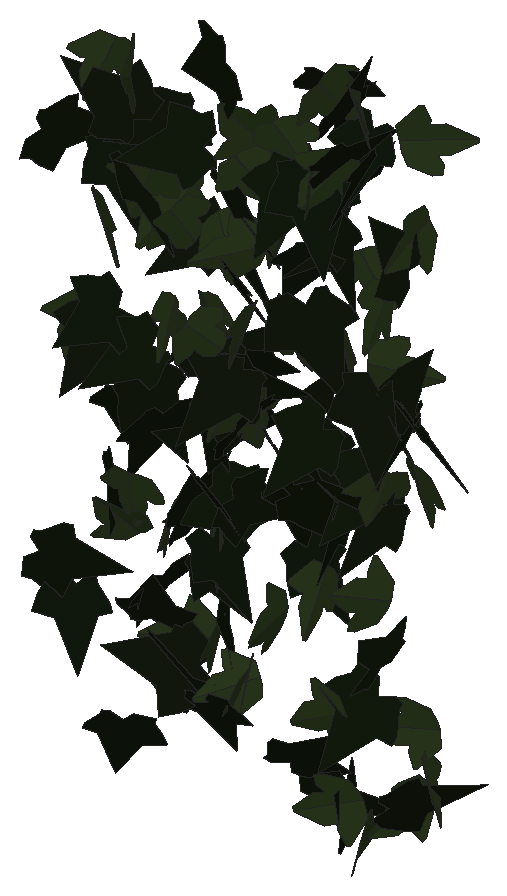
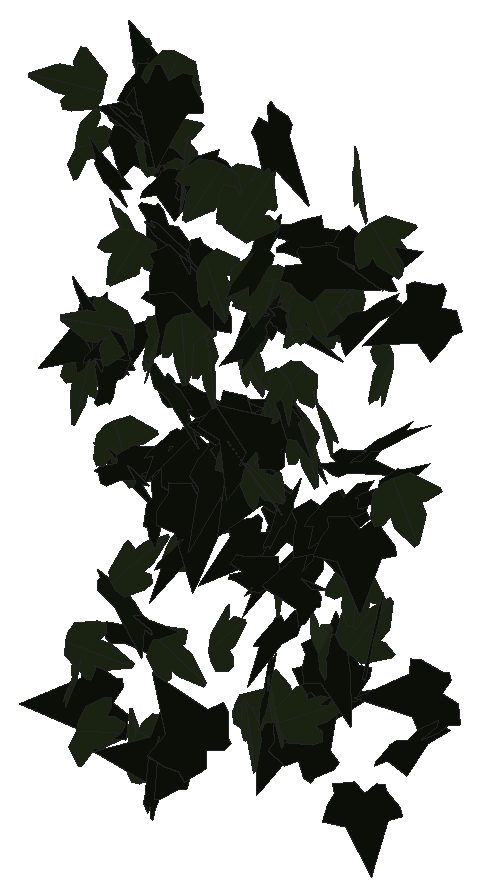
# SketchUp Ruby script. Lengths in inches.
U = 1.inch
M = Sketchup.active_model
def pt(a) = Geom::Point3d.new(a.map { |v| v * U })
def face(e, loops, mat)
  f = e.add_face(loops[0].map { |a| pt(a) })
  loops[1..].each { |l| e.add_face(l.map { |a| pt(a) }).erase! }
  f.material = f.back_material = mat if mat
  f
end
# faces: each face lists its corners as indices into pts; further lists are holes
def faces(e, pts, list, mat = nil) = list.each { |f| face(e, (f[0].is_a?(Array) ? f : [f]).map { |l| l.map { |i| pts[i] } }, mat) }
# xy, xz, yz: faces in a plane at the given z, y or x. An outline is a flat list of corners, or four numbers for a rectangle; further outlines are holes
def ring(l) = l.size == 4 ? [[l[0], l[1]], [l[2], l[1]], [l[2], l[3]], [l[0], l[3]]] : l.each_slice(2).to_a
def flat(e, list, mat, &to3) = list.each { |f| face(e, (f[0].is_a?(Array) ? f : [f]).map { |l| ring(l).map { |u, v| to3.(u, v) } }, mat) }
def xy(e, z, list, mat = nil) = flat(e, list, mat) { |x, y| [x, y, z] }
def xz(e, y, list, mat = nil) = flat(e, list, mat) { |x, z| [x, y, z] }
def yz(e, x, list, mat = nil) = flat(e, list, mat) { |y, z| [x, y, z] }
def lines(e, pts, list) = list.each { |a, b| e.add_line(pt(pts[a]), pt(pts[b])) }
# prism: a flat outline (further loops are holes) pulled along v
def prism(e, loops, v, mat = nil)
  f = face(e, loops, mat); d = Geom::Vector3d.new(v.map { |x| x * U })
  f.pushpull(f.normal.samedirection?(d) ? d.length : -d.length)
end
def box(e, o, s, mat = nil) = prism(e, [[o, [o[0] + s[0], o[1], o[2]], [o[0] + s[0], o[1] + s[1], o[2]], [o[0], o[1] + s[1], o[2]]]], [0, 0, s[2]], mat)
def at(x, y, z, deg = 0) = Geom::Transformation.translation(pt([x, y, z])) * Geom::Transformation.rotation(ORIGIN, Z_AXIS, deg.degrees)
def axes(o, x, y, z) = Geom::Transformation.new([*x, 0, *y, 0, *z, 0, *pt(o).to_a, 1])
def part(name) = M.definitions.add(name)
# library, detail: a bought-in or finely detailed component or shape, given as its bounding box
def library(name, o, s) = part(name).tap { |d| box(d.entities, o, s) }
def detail(e, o, s) = box(e.add_group.entities, o, s)
def put(e, d, t, mat = nil) = e.add_instance(d, t).tap { |i| i.material = mat if mat }
def group(e, t, mat = nil) = e.add_group.tap { |g| g.transformation = t; g.material = mat if mat }.entities
root = M.entities
M.materials.add("efeu1").color = [18, 25, 13]
M.materials.add("efeu2").color = [43, 57, 29]
c1 = part("ivyleaf_9")
p = [[1.54,2.16,1.25],[1.36,2.04,1.19],[-0.21,0.99,0.68],[-0.71,1.11,0.82],[-0.85,0.86,0.67],[-0.8,0.17,0.21],
  [-0.9,-0.01,0.1],[-0.67,-0.16,-0.02],[-0.08,-0.08,-0.05],[-0.03,-0.6,-0.4],[0.65,-0.88,-0.66],[0.83,-0.6,-0.49],
  [1.29,-0.42,-0.43],[1.8125,-0.07,-0.26],[1.21,0.44,0.15]]
faces(c1.entities,p,[[0,1,2,3,4,5,6,7,8,9,10,11,12,13,14]],"efeu1")
c2 = part("ivyleaf_10")
p = [[0,0.5,-0.03],[-0.0625,2.02,-0.43],[-0.19,2.01,-0.46],[-0.54,1.05,-0.29],[-0.52,0.625,-0.18],[-0.83,0.76,-0.28],
  [-1.16,0.64,-0.33],[-1.15,0.33,-0.24],[-0.77,-0.39,0.02],[-0.3,-0.51,0.16],[0.04,-0.48,0.23],[-0.02,2.01,-0.4375],
  [-0.06,2.01,-0.43],[0.04,-0.49,0.23],[0.67,-0.49,0.14],[1.38,0.36,-0.2],[1.375,0.51,-0.24],[0.81,0.65,-0.19],
  [0.62,0.59,-0.15],[0.6,1.09,-0.28],[0.5,1.23,-0.31]]
faces(c2.entities,p,[[0,1,2,3,4,5,6,7,8,9,10],[11,12,0,13,14,15,16,17,18,19,20]],"efeu2")
put(root,c1,axes([588.51,122.66,270.91],[-0.74172,-0.90871,0.06733],[-0.04182,-0.05278,-1.17299],[0.91024,-0.7429,0.00098]))
put(root,c1,axes([580.71,122.18,269.04],[0.81579,-1.023,-0.08756],[-0.04846,0.07335,-1.30842],[1.02559,0.81719,0.00782]))
put(root,c1,axes([589.85,122.54,260.28],[-1.13073,-0.3644,-0.00526],[0.00461,0.00284,-1.188],[0.36441,-1.13074,-0.00129]))
put(root,c2,axes([585.97,122.9,266.96],[0.01657,-0.06122,1.22241],[-0.38228,-1.16162,-0.05299],[1.16271,-0.38105,-0.03485]))
put(root,c2,axes([581.17,121.5625,273.54],[-0.35287,0.47131,1.0792],[-0.97985,0.50742,-0.54198],[-0.65322,-1.01574,0.23001]))
put(root,c2,axes([593.1,122.29,267.33],[1.04365,-0.66297,-0.14136],[-0.12351,0.06921,-1.2364],[0.66653,1.05091,-0.00776]))
put(root,c1,axes([581.53,122.46,249.09],[1.04021,0.12419,0.34433],[-0.34136,-0.04538,1.04759],[0.13215,-1.09478,-0.00437]))
put(root,c1,axes([579.07,123.16,261.7],[-0.65483,-0.64137,0.7681],[-0.23823,-0.79163,-0.86412],[0.97189,-0.62618,0.3057]))
put(root,c2,axes([586.5,121.96,271.31],[-0.751,-0.60655,-0.59353],[0.56348,0.23624,-0.9544],[0.63457,-0.92762,0.14504]))
put(root,c1,axes([583.23,123.04,247.2],[-0.35084,-1.06025,-0.7792],[-0.16835,-0.76362,1.11486],[-1.30496,0.38356,0.06567]))
put(root,c1,axes([580.4,122,244.14],[0.57176,0.723,-0.64102],[-0.37666,-0.51914,-0.9215],[-0.8898,0.68433,-0.02182]))
put(root,c2,axes([594.57,123.05,270.72],[0.10874,0.42943,-1.1541],[-0.22975,-1.13117,-0.44255],[-1.20978,0.25342,-0.01969]))
put(root,c1,axes([584.45,121.9,256.28],[1.01147,-0.09508,-0.43493],[-0.42674,0.10069,-1.01442],[0.1269,1.09641,0.05545]))
put(root,c1,axes([584.8,122.27,253.67],[0.45808,-1.01494,-0.46328],[-0.10905,0.45768,-1.11049],[1.11033,0.46368,0.08207]))
put(root,c2,axes([589.57,122.96,253.28],[-0.21069,-0.89114,0.74896],[0.40849,-0.76932,-0.80046],[1.09005,0.11606,0.44473]))
put(root,c2,axes([590.56,122.79,272.26],[-0.62203,-0.77137,0.76488],[-0.4405,-0.62658,-0.99012],[0.99299,-0.76116,0.03992]))
put(root,c2,axes([581.43,122.43,268.875],[-0.95805,-0.57927,0.43833],[-0.39346,-0.19604,-1.11906],[0.61064,-1.03516,-0.03335]))
put(root,c2,axes([590.67,122.49,247.87],[-0.44719,-0.10103,1.05054],[-1.00704,-0.30051,-0.45757],[0.31575,-1.1015,0.02848]))
put(root,c1,axes([594.55,122.03,269.44],[-0.82004,0.10315,-0.88856],[-0.89316,-0.02771,0.82107],[0.04951,1.20882,0.09464]))
put(root,c2,axes([591.71,122.8,241.96],[0.34312,-1.07913,-0.40514],[0.17503,-0.36903,1.13118],[-1.13931,-0.38169,0.05177]))
put(root,c1,axes([585.45,122.99,261.21],[-1.3014,-0.34703,-0.02695],[0.01969,0.03073,-1.34665],[0.34752,-1.30131,-0.02462]))
put(root,c2,axes([584.18,123.04,253.04],[-0.37858,0.38595,-0.95882],[0.44707,-0.8595,-0.5225],[-0.93189,-0.56913,0.13886]))
put(root,c1,axes([594.21,122.91,262.05],[-0.78595,0.35453,-0.68866],[0.54325,-0.44703,-0.85013],[-0.55212,-0.94453,0.14386]))
put(root,c1,axes([576.48,121.97,250.41],[0.42857,0.21806,-1.12222],[0.56145,1.00384,0.40947],[0.99584,-0.65981,0.2521]))
put(root,c1,axes([589.29,122.91,271.21],[-0.16246,-1.28596,-0.40789],[0.03143,0.40712,-1.29604],[1.34873,-0.16439,-0.01893]))
put(root,c2,axes([583.89,122.11,262.95],[-0.34525,-0.70898,-0.784],[0.52502,0.60081,-0.77452],[0.91742,-0.61063,0.14821]))
put(root,c1,axes([580.72,123.25,260.55],[-0.89333,-0.43925,0.45376],[-0.34698,-0.31541,-0.98843],[0.52768,-0.95103,0.11824]))
put(root,c1,axes([584.48,122.18,246.4],[0.96419,0.41931,-0.38004],[-0.35414,-0.13853,-1.05134],[-0.4414,1.02709,0.01335]))
put(root,c1,axes([585.14,122.32,266.17],[1.06845,-0.15647,-0.28734],[-0.28332,0.04837,-1.07983],[0.16364,1.10536,0.00658]))
put(root,c1,axes([592.05,123.23,248.71],[-1.09626,-0.5986,0.03158],[-0.02807,-0.01448,-1.24904],[0.59877,-1.09662,-0.00075]))
put(root,c2,axes([579.9,123.09,252.21],[-0.88437,-0.18792,-0.61587],[-0.50487,-0.44705,0.86138],[-0.39965,0.98059,0.27467]))
put(root,c2,axes([585.83,123,263.85],[0.31886,-1.02934,0.29924],[0.06734,-0.29234,-1.07739],[1.06984,0.32519,-0.02138]))
put(root,c2,axes([580.4,122.6,254.65],[-1.07219,-0.16162,0.08184],[-0.07979,-0.01977,-1.08427],[0.16264,-1.07513,0.00763]))
put(root,c1,axes([583.14,123.39,270.29],[-0.7313,-0.24912,0.86653],[-0.7634,-0.42258,-0.76575],[0.47974,-1.05218,0.10239]))
put(root,c1,axes([577.12,123.14,248.49],[-0.11856,-1.14911,-0.19067],[0.02311,0.1893,-1.1552],[1.16459,-0.12074,0.00351]))
put(root,c2,axes([585.49,123.36,247.16],[-0.38609,0.02502,0.98744],[-0.50808,-0.91421,-0.1755],[0.84706,-0.53695,0.34481]))
put(root,c1,axes([581.87,122.6,250.875],[-0.29585,1.01359,-0.39261],[0.12946,-0.37114,-1.05571],[-1.07923,-0.32237,-0.01901]))
put(root,c1,axes([583.02,122.98,245.56],[0.7891,-0.43198,0.89447],[-0.78525,0.42832,0.8996],[-0.60833,-1.11324,-0.00097]))
put(root,c1,axes([592.2,123.26,262.43],[-0.25174,-1.27421,-0.24221],[0.06913,0.2332,-1.29865],[1.29518,-0.26011,0.02224]))
put(root,c1,axes([590.57,121.93,272.55],[0.11115,1.07817,-0.5978],[0.07088,0.59364,1.08385],[1.23077,-0.13156,-0.00844]))
put(root,c2,axes([582.71,122.49,267.41],[-0.48849,-0.88996,-0.6184],[0.39972,0.48254,-1.01018],[1.00732,-0.62306,0.10096]))
put(root,c1,axes([578.16,123.73,260.45],[-0.55641,-1.02095,0.4111],[-0.12253,-0.40033,-1.16003],[1.09377,-0.56422,0.07918]))
put(root,c2,axes([582.08,123.52,267.59],[-0.57498,-0.71135,0.88246],[-0.2973,-0.86022,-0.88713],[1.09379,-0.60775,0.22276]))
put(root,c2,axes([591.6,122.59,275.77],[-0.78903,0.82604,0.16505],[-0.09999,0.1327,-1.14217],[-0.83641,-0.79511,-0.01915]))
put(root,c2,axes([590.86,122.98,243.78],[0.50999,0.05024,-1.12526],[-1.12588,0.05956,-0.50762],[0.03357,1.234,0.07032]))
put(root,c1,axes([588.93,122.86,265.31],[-0.45093,-0.7202,-1.03942],[0.51545,0.90301,-0.84929],[1.15473,-0.68433,-0.02679]))
put(root,c2,axes([589.45,122.42,271.73],[0.50004,-0.76891,-0.81576],[-0.14598,0.84097,-0.88215],[1.11147,0.45638,0.25114]))
put(root,c2,axes([594.69,122.78,259.85],[-1.09015,0.52447,0.12319],[-0.11065,0.05415,-1.20975],[-0.52725,-1.09575,-0.00082]))
put(root,c1,axes([588.625,122.46,256.99],[0.53694,0.47109,-1.0485],[0.6045,0.86857,0.69981],[0.97767,-0.79576,0.14313]))
put(root,c1,axes([590.36,122.94,274.22],[0.30107,1.11029,0.52357],[-0.16912,-0.49643,1.14998],[1.21584,-0.34399,0.03031]))
put(root,c2,axes([581.7,123.26,262.5625],[0.89512,-0.62561,0.1387],[0.11377,-0.07933,-1.09207],[0.63062,0.90232,0.00015]))
put(root,c2,axes([590.05,122.6,275.6875],[-0.42358,-0.91674,-0.75887],[0.35652,0.67076,-1.00931],[1.13543,-0.55262,0.03382]))
put(root,c1,axes([593.89,123.07,262.13],[1.09995,-0.65109,0.07127],[0.07191,-0.01841,-1.27803],[0.65102,1.1021,0.02075]))
put(root,c1,axes([581.5,123.11,257.77],[-0.1376,1.09253,-0.72485],[0.06561,-0.72218,-1.10096],[-1.30948,-0.15099,0.02101]))
put(root,c1,axes([584.75,122.85,274.85],[0.03118,0.19742,-1.3483],[-1.33653,-0.25848,-0.06876],[-0.26564,1.32366,0.18767]))
put(root,c1,axes([591.6875,123.6,272.66],[-0.52583,0.60273,-0.83521],[0.43475,-0.72025,-0.79347],[-0.93373,-0.67477,0.1009]))
put(root,c2,axes([586.45,124.1,250.16],[0.0163,0.01032,1.20059],[0.50487,-1.08944,0.00251],[1.08933,0.50477,-0.01913]))
put(root,c2,axes([582.59,123.95,247.91],[0.11599,0.28254,1.15628],[-0.42683,-1.07462,0.3054],[1.11114,-0.4423,-0.00339]))
put(root,c2,axes([578.27,123.27,266.08],[-0.8312,0.83154,-0.42194],[0.30519,-0.2915,-1.17569],[-0.88111,-0.88541,-0.00919]))
put(root,c1,axes([583.58,123.63,266.52],[-1.08853,-0.02079,0.21967],[-0.21903,-0.03195,-1.08839],[0.02669,-1.11002,0.02721]))
put(root,c1,axes([587.95,123.25,244.46],[1.09431,0.63073,-0.20183],[0.17273,0.10447,1.26306],[0.63931,-1.10785,0.0042]))
put(root,c2,axes([584.52,123.1,267.33],[0.37719,1.09901,0.16166],[0.03937,0.15739,-1.16186],[-1.11014,0.37899,0.01372]))
put(root,c1,axes([584.55,123.28,269.18],[1.09148,-0.77338,-0.13015],[-0.10588,0.07568,-1.3377],[0.77707,1.09661,0.00054]))
put(root,c1,axes([576.16,122.46,269.04],[0.09721,0.40459,-1.15688],[-0.14904,1.1558,0.39168],[1.21649,0.10928,0.14044]))
put(root,c1,axes([578.15,124.25,253.4],[0.3939,-0.34619,-1.19939],[1.10372,-0.49105,0.50421],[-0.58327,-1.163,0.14414]))
put(root,c1,axes([588.82,123.45,267.52],[0.14651,0.87061,-0.72867],[-0.23464,-0.69563,-0.87832],[-1.1108,0.26178,0.08942]))
put(root,c1,axes([589.51,123.68,268.84],[-0.48933,-0.2087,-1.06709],[1.00465,0.36075,-0.53125],[0.41584,-1.11713,0.0278]))
put(root,c1,axes([588.97,123.47,259.12],[0.36284,-0.99249,-0.57538],[-0.08185,0.57954,-1.05128],[1.14429,0.35616,0.10725]))
put(root,c1,axes([579.59,123.48,270.41],[-0.1378,0.22071,1.22906],[-1.17195,0.404,-0.20395],[-0.43106,-1.16891,0.16157]))
put(root,c1,axes([582.78,122.5,253.78],[0.1554,0.23556,1.2837],[0.48368,1.19032,-0.27698],[-1.2122,0.50515,0.05405]))
put(root,c1,axes([583.03,124.34,257.18],[0.10987,-0.70699,0.90466],[0.19064,-0.88494,-0.71474],[1.13221,0.21762,0.03256]))
put(root,c1,axes([591.95,124.15,260.92],[0.37772,-0.59464,0.91033],[0.43918,-0.79815,-0.70359],[0.99469,0.57821,-0.03502]))
put(root,c1,axes([578.85,123.85,268.51],[0.05607,-1.19416,-0.39132],[0.07719,0.39424,-1.19202],[1.25427,0.02912,0.09085]))
put(root,c2,axes([588.76,123.59,264.16],[-0.24705,-1.12116,-0.09841],[0.02227,0.09586,-1.14806],[1.12526,-0.24805,0.00112]))
put(root,c1,axes([580.48,123.37,258.85],[0.32041,-0.95034,-0.85727],[-0.29122,0.80641,-1.00281],[1.2463,0.43275,-0.01392]))
put(root,c1,axes([583.09,123.45,262.1],[-0.71457,0.84188,-0.07063],[0.04467,-0.05472,-1.10425],[-0.84365,-0.71596,0.00135]))
put(root,c1,axes([589.78,124.26,256.01],[-0.28989,0.08558,-1.09684],[0.85588,-0.69515,-0.28045],[-0.69127,-0.89658,0.11275]))
put(root,c2,axes([585.26,123.55,247.15],[0.30776,-1.12767,-0.29822],[-0.08336,0.28638,-1.1689],[1.16346,0.31882,-0.00487]))
put(root,c2,axes([585.69,123.46,259.57],[-0.39783,-1.11946,-0.31869],[0.08398,0.30831,-1.18782],[1.16091,-0.40593,-0.02328]))
put(root,c1,axes([592.2,124,257.04],[-1.20961,0.01465,-0.26376],[0.26318,-0.03981,-1.20917],[-0.02279,-1.23739,0.03578]))
put(root,c1,axes([592.55,123.57,261.7],[-0.52799,0.57376,0.97393],[0.66918,-0.70767,0.77969],[0.91101,0.85236,-0.00826]))
put(root,c2,axes([578.05,124.12,272.62],[-0.59175,-0.8195,0.54675],[-0.09231,-0.58888,-0.98255],[0.98082,-0.54985,0.2374]))
put(root,c2,axes([591.99,123.88,258.125],[-0.51904,-0.99487,0.25396],[-0.12845,-0.21941,-1.12206],[1.0187,-0.53456,-0.01209]))
put(root,c1,axes([589.29,123.33,243.2],[0.68238,-0.01309,1.00643],[1.00615,-0.02398,-0.68251],[0.0272,1.21572,-0.00263]))
put(root,c2,axes([583.46,123.69,263.18],[-0.89992,0.46871,-0.43556],[0.36506,-0.24119,-1.01382],[-0.52549,-0.97026,0.04161]))
put(root,c1,axes([588.53,123.55,254],[0.40999,-0.90524,-0.67299],[-0.19806,0.64717,-0.99117],[1.11047,0.44964,0.07169]))
put(root,c1,axes([591.1875,124.08,273.5],[-1.00706,-0.31467,-0.45748],[0.44288,0.11626,-1.0549],[0.3349,-1.09997,0.01937]))
put(root,c1,axes([583.61,124.61,248.6],[-0.06943,-0.09793,1.39313],[0.10327,-1.3914,-0.09266],[1.39275,0.09829,0.07632]))
put(root,c1,axes([587.09,123.22,258.21],[1.06151,-0.02891,-0.80604],[-0.79637,0.17363,-1.05499],[0.12785,1.3215,0.12098]))
put(root,c2,axes([577.01,124.05,260.7],[-0.7195,-0.90514,0.4233],[-0.16383,-0.4077,-1.15025],[0.9857,-0.72845,0.1178]))
put(root,c2,axes([585.04,124.43,271.04],[-0.5949,-0.7157,-0.81523],[-0.47165,-0.66665,0.92944],[-0.97692,0.75768,0.04771]))
put(root,c1,axes([593.29,122.86,244.45],[0.18674,0.88779,-0.93503],[0.18639,0.91628,0.90721],[1.27582,-0.26381,0.00432]))
put(root,c2,axes([583.74,123.84,248.89],[0.46508,-1.09845,-0.15462],[-0.04069,0.15065,-1.19266],[1.10853,0.46638,0.02109]))
put(root,c2,axes([584.23,124.41,259.31],[-0.02692,-0.8716,0.71638],[0.0472,-0.71683,-0.87037],[1.12723,0.0092,0.05355]))
put(root,c2,axes([581.53,124.03,268.32],[-0.64095,-0.81554,0.40318],[-0.26758,-0.30239,-1.03704],[0.86952,-0.69421,-0.02193]))
put(root,c2,axes([593.1,124.57,244.04],[0.19381,0.4703,-1.1324],[-0.53053,-1.00142,-0.5067],[-1.10546,0.56306,0.04465]))
put(root,c1,axes([589.65,124.07,268.68],[-1.13663,0.1888,-0.00332],[0.00363,0.00163,-1.1522],[-0.18879,-1.13664,-0.00221]))
put(root,c1,axes([585.26,123.05,255.36],[0.15704,0.04249,-1.1026],[-0.30636,1.0716,-0.00234],[1.06003,0.30341,0.16267]))
put(root,c2,axes([594.35,123.7,246.09],[-0.58262,0.99678,-0.04156],[0.02109,-0.03581,-1.15456],[-0.99742,-0.583,-0.00014]))
put(root,c1,axes([579.43,123.58,257.73],[0.64302,0.74994,-0.59671],[-0.41526,-0.42959,-0.98739],[-0.86373,0.76484,0.03049]))
put(root,c2,axes([590.99,124.65,252.1875],[-0.01448,0.54847,1.09855],[0.04352,-1.0977,0.54862],[1.22708,0.04541,-0.00649]))
put(root,c2,axes([580.72,124.65,252.29],[-0.29716,0.049,-1.06746],[0.24003,-1.07659,-0.11624],[-1.04128,-0.26215,0.27784]))
put(root,c1,axes([584.54,123.56,260.36],[0.55146,0.37113,-0.99817],[0.74094,0.67368,0.65982],[0.76492,-0.92012,0.08049]))
put(root,c1,axes([583.45,123.65,252.01],[0.34615,-0.72376,-0.75846],[-0.3362,0.67991,-0.80224],[0.993,0.48249,-0.00722]))
put(root,c2,axes([589.92,124.14,263.45],[-0.58695,0.82154,-0.63829],[0.34648,-0.53667,-1.00935],[-0.98096,-0.68111,0.02541]))
put(root,c1,axes([589.59,124.65,242.04],[0.02528,0.223,1.25674],[-0.14624,-1.24821,0.22442],[1.26797,-0.1484,0.00083]))
put(root,c1,axes([587.95,123.57,256.16],[0.87441,0.59143,-0.70397],[-0.59244,-0.38051,-1.05555],[-0.70313,1.05612,0.01392]))
put(root,c2,axes([582.4,123.68,261.39],[-0.76466,0.17773,0.774],[-0.7651,0.12307,-0.78413],[-0.21282,-1.08104,0.03798]))
put(root,c1,axes([584.71,124.47,254.45],[-0.92697,-0.17104,0.70289],[-0.67795,-0.19319,-0.94109],[0.25237,-1.14717,0.05369]))
put(root,c2,axes([586.94,123.8,272.15],[-0.93327,-0.47595,-0.52659],[0.52704,0.11802,-1.04073],[0.47545,-1.06506,0.11999]))
put(root,c2,axes([593.8,124.09,247.62],[0.2518,-0.03689,-1.16536],[-1.16559,0.02133,-0.25253],[0.02864,1.19206,-0.03154]))
put(root,c1,axes([583.58,123.53,260.24],[-0.16789,-0.03446,1.18247],[1.17015,0.1705,0.17111],[-0.17367,1.18209,0.00979]))
put(root,c2,axes([587.55,123.65,263.61],[-0.81688,0.37823,0.76082],[-0.73246,0.22138,-0.89649],[-0.43059,-1.09414,0.08162]))
put(root,c1,axes([585.39,122.96,258.62],[0.29643,1.14778,0.66283],[0.17018,0.64062,-1.18543],[-1.31445,0.34178,-0.00399]))
put(root,c1,axes([589.55,123.61,275.56],[0.77971,0.81246,-0.47219],[-0.35452,-0.3139,-1.12552],[-0.87027,0.85579,0.03545]))
put(root,c1,axes([591.01,124.91,257.6],[-0.8077,-0.88905,0.38187],[-0.26043,-0.27932,-1.20115],[0.93189,-0.84863,-0.0047]))
put(root,c2,axes([586.65,124.39,268.03],[0.08571,-1.15597,0.21565],[0.00734,-0.21569,-1.15911],[1.17589,0.0856,-0.00848]))
put(root,c1,axes([583.98,124.23,266.21],[0.91351,-0.89137,-0.01362],[-0.00829,0.011,-1.27633],[0.89143,0.91354,0.00208]))
put(root,c1,axes([589.58,123.68,261.46],[-0.60686,0.92777,0.43428],[-0.27629,0.33782,-1.10778],[-0.98642,-0.6654,0.0431]))
put(root,c1,axes([592.09,123.4375,250.14],[-0.28946,1.00279,0.71441],[-0.43602,0.60284,-1.02285],[-1.15146,-0.48037,0.20773]))
put(root,c2,axes([590.98,124.11,267.63],[-0.92374,-0.40249,-0.4536],[0.50076,-0.04007,-0.98421],[0.34204,-1.02832,0.2159]))
put(root,c1,axes([585.13,123.65,261.32],[0.85124,0.83001,-0.31115],[-0.23683,-0.20274,-1.18875],[-0.85419,0.88335,0.01952]))
put(root,c1,axes([581.33,124.75,270.35],[-0.12544,-0.25103,-1.12163],[-0.52867,-0.98925,0.28053],[-1.02058,0.54329,-0.00746]))
put(root,c1,axes([585.23,123.56,258.66],[-1.03041,0.36685,-0.63807],[-0.60169,0.21238,1.09377],[0.42389,1.19322,0.0015]))
put(root,c2,axes([591.89,124.02,263.29],[-0.09085,0.0383,-1.23942],[1.23869,0.06027,-0.08894],[0.05734,-1.24128,-0.04256]))
put(root,c2,axes([593.67,123.74,274.03],[-0.19531,-0.12717,1.20138],[0.89115,0.80652,0.23025],[-0.81568,0.91159,-0.03611]))
